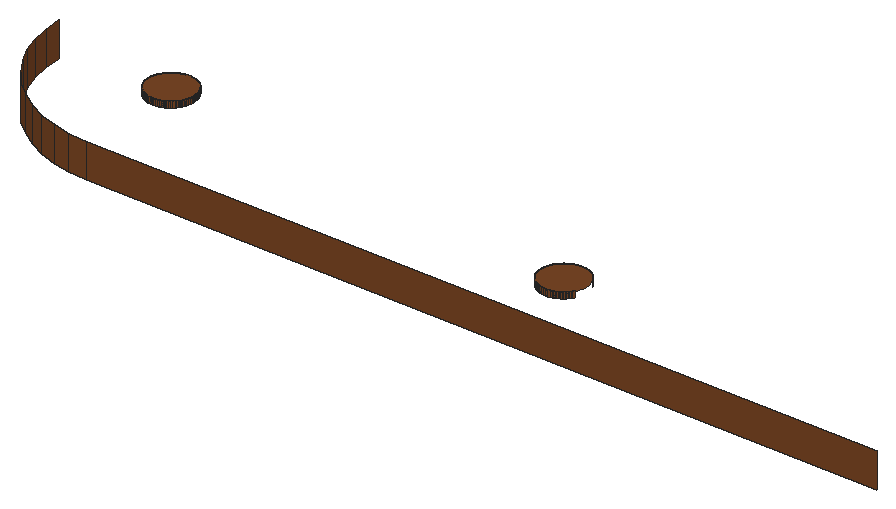
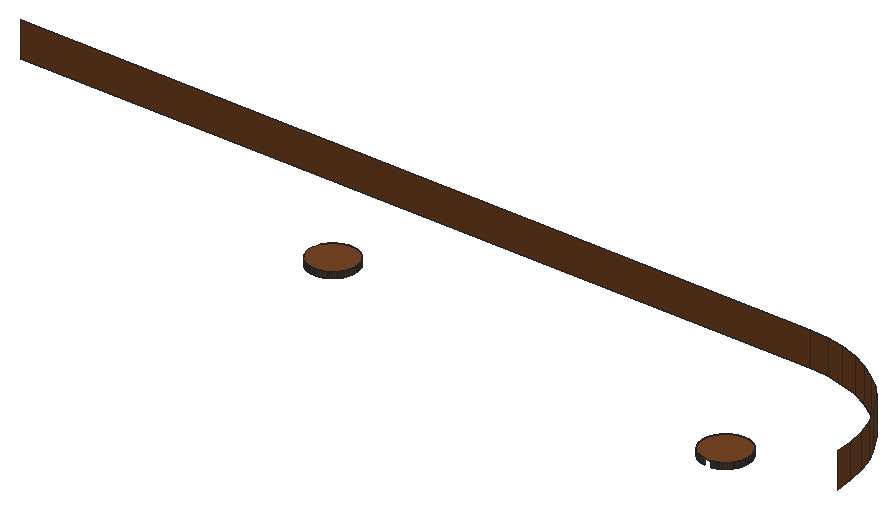
# SketchUp Ruby script. Lengths in inches.
U = 1.inch
M = Sketchup.active_model
def pt(a) = Geom::Point3d.new(a.map { |v| v * U })
def face(e, loops, mat)
  f = e.add_face(loops[0].map { |a| pt(a) })
  loops[1..].each { |l| e.add_face(l.map { |a| pt(a) }).erase! }
  f.material = f.back_material = mat if mat
  f
end
# faces: each face lists its corners as indices into pts; further lists are holes
def faces(e, pts, list, mat = nil) = list.each { |f| face(e, (f[0].is_a?(Array) ? f : [f]).map { |l| l.map { |i| pts[i] } }, mat) }
# xy, xz, yz: faces in a plane at the given z, y or x. An outline is a flat list of corners, or four numbers for a rectangle; further outlines are holes
def ring(l) = l.size == 4 ? [[l[0], l[1]], [l[2], l[1]], [l[2], l[3]], [l[0], l[3]]] : l.each_slice(2).to_a
def flat(e, list, mat, &to3) = list.each { |f| face(e, (f[0].is_a?(Array) ? f : [f]).map { |l| ring(l).map { |u, v| to3.(u, v) } }, mat) }
def xy(e, z, list, mat = nil) = flat(e, list, mat) { |x, y| [x, y, z] }
def xz(e, y, list, mat = nil) = flat(e, list, mat) { |x, z| [x, y, z] }
def yz(e, x, list, mat = nil) = flat(e, list, mat) { |y, z| [x, y, z] }
def lines(e, pts, list) = list.each { |a, b| e.add_line(pt(pts[a]), pt(pts[b])) }
# prism: a flat outline (further loops are holes) pulled along v
def prism(e, loops, v, mat = nil)
  f = face(e, loops, mat); d = Geom::Vector3d.new(v.map { |x| x * U })
  f.pushpull(f.normal.samedirection?(d) ? d.length : -d.length)
end
def box(e, o, s, mat = nil) = prism(e, [[o, [o[0] + s[0], o[1], o[2]], [o[0] + s[0], o[1] + s[1], o[2]], [o[0], o[1] + s[1], o[2]]]], [0, 0, s[2]], mat)
def at(x, y, z, deg = 0) = Geom::Transformation.translation(pt([x, y, z])) * Geom::Transformation.rotation(ORIGIN, Z_AXIS, deg.degrees)
def axes(o, x, y, z) = Geom::Transformation.new([*x, 0, *y, 0, *z, 0, *pt(o).to_a, 1])
def part(name) = M.definitions.add(name)
# library, detail: a bought-in or finely detailed component or shape, given as its bounding box
def library(name, o, s) = part(name).tap { |d| box(d.entities, o, s) }
def detail(e, o, s) = box(e.add_group.entities, o, s)
def put(e, d, t, mat = nil) = e.add_instance(d, t).tap { |i| i.material = mat if mat }
def group(e, t, mat = nil) = e.add_group.tap { |g| g.transformation = t; g.material = mat if mat }.entities
root = M.entities
M.materials.add("[Wood Veneer 01]3").color = [120, 70, 37]
xy(root,118.5,[[109.4,34,109.24,34.02,109.15,34.03,108.91,34.09,108.67,34.18,108.6,34.21,108.52,34.25,108.45,34.3,108.38,34.34,108.3125,34.39,108.25,34.44,108.18,34.5,108.12,34.55,108.0625,34.61,108,34.67,107.95,34.74,107.9,34.8,107.8,34.94,107.76,35.01,107.72,35.09,107.68,35.16,107.59,35.4,107.53,35.64,107.51,35.8,107.5,35.89,107.5,36.14,107.51,36.22,107.52,36.31,107.6,36.63,107.66,36.79,107.7,36.86,107.73,36.9375,107.77,37.01,107.97,37.29,108.02,37.35,108.14,37.47,108.2,37.52,108.27,37.58,108.34,37.625,108.4,37.67,108.48,37.72,108.55,37.76,108.625,37.8,108.7,37.83,108.94,37.92,109.1,37.96,109.18,37.97,109.26,37.99,109.35,37.99,109.43,38,109.6,38,109.76,37.98,109.85,37.97,110.09,37.91,110.33,37.82,110.4,37.79,110.48,37.75,110.55,37.7,110.62,37.66,110.6875,37.61,110.75,37.56,110.82,37.5,110.88,37.45,110.9375,37.39,111,37.33,111.05,37.26,111.1,37.2,111.2,37.06,111.24,36.99,111.28,36.91,111.32,36.84,111.41,36.6,111.47,36.36,111.49,36.2,111.5,36.11,111.5,35.86,111.49,35.78,111.48,35.69,111.4,35.37,111.34,35.21,111.3,35.14,111.27,35.0625,111.23,34.99,111.03,34.71,110.98,34.65,110.86,34.53,110.8,34.48,110.73,34.42,110.66,34.375,110.6,34.33,110.52,34.28,110.45,34.24,110.375,34.2,110.3,34.17,110.06,34.08,109.9,34.04,109.82,34.03,109.74,34.01,109.65,34.01,109.57,34],[71.9,38,71.74,38.02,71.65,38.03,71.41,38.09,71.17,38.18,71.1,38.21,71.02,38.25,70.95,38.3,70.88,38.34,70.8125,38.39,70.75,38.44,70.68,38.5,70.62,38.55,70.5625,38.61,70.5,38.67,70.45,38.74,70.4,38.8,70.3,38.94,70.26,39.01,70.22,39.09,70.18,39.16,70.09,39.4,70.03,39.64,70.01,39.8,70,39.89,70,40.14,70.01,40.22,70.02,40.31,70.1,40.63,70.16,40.79,70.2,40.86,70.23,40.9375,70.27,41.01,70.47,41.29,70.52,41.35,70.64,41.47,70.7,41.52,70.77,41.58,70.84,41.625,70.9,41.67,70.98,41.72,71.05,41.76,71.125,41.8,71.2,41.83,71.44,41.92,71.6,41.96,71.68,41.97,71.76,41.99,71.85,41.99,71.93,42,72.1,42,72.26,41.98,72.35,41.97,72.59,41.91,72.83,41.82,72.9,41.79,72.98,41.75,73.05,41.7,73.12,41.66,73.1875,41.61,73.25,41.56,73.32,41.5,73.38,41.45,73.4375,41.39,73.5,41.33,73.55,41.26,73.6,41.2,73.7,41.06,73.74,40.99,73.78,40.91,73.82,40.84,73.91,40.6,73.97,40.36,73.99,40.2,74,40.11,74,39.86,73.99,39.78,73.98,39.69,73.9,39.37,73.84,39.21,73.8,39.14,73.77,39.0625,73.73,38.99,73.53,38.71,73.48,38.65,73.36,38.53,73.3,38.48,73.23,38.42,73.16,38.375,73.1,38.33,73.02,38.28,72.95,38.24,72.875,38.2,72.8,38.17,72.56,38.08,72.4,38.04,72.32,38.03,72.24,38.01,72.15,38.01,72.07,38]],"[Wood Veneer 01]3")
xz(root,27,[[75,118,144,121]],"[Wood Veneer 01]3")
xz(root,34,[[109.4,118,109.49,118.5],[109.49,118,109.57,118.5]],"[Wood Veneer 01]3")
xz(root,34.01,[[109.65,118,109.74,118.5]],"[Wood Veneer 01]3")
xz(root,37.99,[[109.26,118,109.35,118.5]],"[Wood Veneer 01]3")
xz(root,38,[[71.9,118,71.99,118.5],[71.99,118,72.07,118.5],[109.43,118,109.51,118.5],[109.51,118,109.6,118.5]],"[Wood Veneer 01]3")
xz(root,38.01,[[72.15,118,72.24,118.5]],"[Wood Veneer 01]3")
yz(root,70,[[39.89,118,39.97,118.5],[39.97,118,40.06,118.5],[40.06,118,40.14,118.5]],"[Wood Veneer 01]3")
yz(root,74,[[39.86,118,39.94,118.5],[39.94,118,40.03,118.5],[40.03,118,40.11,118.5]],"[Wood Veneer 01]3")
yz(root,107.5,[[35.89,118,35.97,118.5],[35.97,118,36.06,118.5],[36.06,118,36.14,118.5]],"[Wood Veneer 01]3")
p = [[75,27,121],[73.43,27.1,121],[73.43,27.1,118],[75,27,118],[71.89,27.41,121],[71.89,27.41,118],
  [70.41,27.91,121],[70.41,27.91,118],[69,28.61,121],[69,28.61,118],[67.69,29.48,121],[67.69,29.48,118],
  [66.51,30.51,121],[66.51,30.51,118],[65.48,31.69,121],[65.48,31.69,118],[64.61,33,121],[64.61,33,118],
  [63.91,34.41,121],[63.91,34.41,118],[109.07,34.05,118],[108.99,34.07,118],[108.99,34.07,118.5],[109.07,34.05,118.5],
  [109.15,34.03,118],[109.15,34.03,118.5],[109.32,34.01,118],[109.24,34.02,118],[109.24,34.02,118.5],[109.32,34.01,118.5],
  [109.4,34,118],[109.4,34,118.5],[109.65,34.01,118],[109.57,34,118],[109.57,34,118.5],[109.65,34.01,118.5],
  [109.82,34.03,118],[109.74,34.01,118],[109.74,34.01,118.5],[109.82,34.03,118.5],[109.9,34.04,118],[109.9,34.04,118.5],
  [109.98,34.06,118],[109.98,34.06,118.5],[108.75,34.15,118],[108.67,34.18,118],[108.67,34.18,118.5],[108.75,34.15,118.5],
  [108.91,34.09,118],[108.83,34.12,118],[108.83,34.12,118.5],[108.91,34.09,118.5],[110.06,34.08,118],[110.06,34.08,118.5],
  [110.14,34.11,118],[110.14,34.11,118.5],[110.22,34.14,118],[110.22,34.14,118.5],[110.3,34.17,118],[110.3,34.17,118.5],
  [108.6,34.21,118],[108.52,34.25,118],[108.52,34.25,118.5],[108.6,34.21,118.5],[110.375,34.2,118],[110.375,34.2,118.5],
  [110.45,34.24,118],[110.45,34.24,118.5],[110.52,34.28,118],[110.52,34.28,118.5],[108.38,34.34,118],[108.3125,34.39,118],
  [108.3125,34.39,118.5],[108.38,34.34,118.5],[108.45,34.3,118],[108.45,34.3,118.5],[110.6,34.33,118],[110.6,34.33,118.5],
  [110.66,34.375,118],[110.66,34.375,118.5],[63.41,35.89,121],[63.41,35.89,118],[108.25,34.44,118],[108.25,34.44,118.5],
  [108.18,34.5,118],[108.18,34.5,118.5],[110.73,34.42,118],[110.73,34.42,118.5],[110.8,34.48,118],[110.8,34.48,118.5],
  [108.12,34.55,118],[108.12,34.55,118.5],[110.86,34.53,118],[110.86,34.53,118.5],[110.92,34.59,118],[110.92,34.59,118.5],
  [108.0625,34.61,118],[108,34.67,118],[108,34.67,118.5],[108.0625,34.61,118.5],[110.98,34.65,118],[110.98,34.65,118.5],
  [107.95,34.74,118],[107.9,34.8,118],[107.9,34.8,118.5],[107.95,34.74,118.5],[111.03,34.71,118],[111.03,34.71,118.5],
  [111.08,34.78,118],[111.08,34.78,118.5],[107.85,34.87,118],[107.85,34.87,118.5],[111.13,34.85,118],[111.13,34.85,118.5],
  [111.18,34.92,118],[111.18,34.92,118.5],[107.8,34.94,118],[107.8,34.94,118.5],[107.76,35.01,118],[107.76,35.01,118.5],
  [111.23,34.99,118],[111.23,34.99,118.5],[107.72,35.09,118],[107.72,35.09,118.5],[107.68,35.16,118],[107.68,35.16,118.5],
  [107.65,35.24,118],[107.62,35.32,118],[107.62,35.32,118.5],[107.65,35.24,118.5],[107.59,35.4,118],[107.59,35.4,118.5],
  [107.57,35.48,118],[107.57,35.48,118.5],[107.55,35.56,118],[107.55,35.56,118.5],[107.53,35.64,118],[107.53,35.64,118.5],
  [107.52,35.72,118],[107.52,35.72,118.5],[107.51,35.8,118],[107.51,35.8,118.5],[107.5,35.89,118],[107.5,35.89,118.5],
  [63.1,37.43,121],[63.1,37.43,118],[107.5,36.14,118],[107.51,36.22,118],[107.51,36.22,118.5],[107.5,36.14,118.5],
  [107.52,36.31,118],[107.52,36.31,118.5],[107.54,36.39,118],[107.54,36.39,118.5],[107.56,36.47,118],[107.56,36.47,118.5],
  [107.58,36.55,118],[107.58,36.55,118.5],[107.6,36.63,118],[107.6,36.63,118.5],[107.63,36.71,118],[107.63,36.71,118.5],
  [107.66,36.79,118],[107.66,36.79,118.5],[107.7,36.86,118],[107.7,36.86,118.5],[107.73,36.9375,118],[107.73,36.9375,118.5],
  [107.77,37.01,118],[107.77,37.01,118.5],[107.82,37.08,118],[107.82,37.08,118.5],[111.2,37.06,118],[111.24,36.99,118],
  [111.24,36.99,118.5],[111.2,37.06,118.5],[107.87,37.15,118],[107.87,37.15,118.5],[111.1,37.2,118],[111.15,37.13,118],
  [111.15,37.13,118.5],[111.1,37.2,118.5],[107.92,37.22,118],[107.92,37.22,118.5],[107.97,37.29,118],[107.97,37.29,118.5],
  [111.05,37.26,118],[111.05,37.26,118.5],[108.02,37.35,118],[108.02,37.35,118.5],[108.08,37.41,118],[108.08,37.41,118.5],
  [110.9375,37.39,118],[111,37.33,118],[111,37.33,118.5],[110.9375,37.39,118.5],[63,39,121],[63,39,118],
  [108.14,37.47,118],[108.14,37.47,118.5],[110.82,37.5,118],[110.88,37.45,118],[110.88,37.45,118.5],[110.82,37.5,118.5],
  [108.2,37.52,118],[108.2,37.52,118.5],[108.27,37.58,118],[108.27,37.58,118.5],[110.75,37.56,118],[110.75,37.56,118.5],
  [108.34,37.625,118],[108.34,37.625,118.5],[108.4,37.67,118],[108.4,37.67,118.5],[110.62,37.66,118],[110.6875,37.61,118],
  [110.6875,37.61,118.5],[110.62,37.66,118.5],[108.48,37.72,118],[108.48,37.72,118.5],[108.55,37.76,118],[108.55,37.76,118.5],
  [110.4,37.79,118],[110.48,37.75,118],[110.48,37.75,118.5],[110.4,37.79,118.5],[110.55,37.7,118],[110.55,37.7,118.5],
  [108.625,37.8,118],[108.625,37.8,118.5],[108.7,37.83,118],[108.7,37.83,118.5],[108.78,37.86,118],[108.78,37.86,118.5],
  [110.25,37.85,118],[110.33,37.82,118],[110.33,37.82,118.5],[110.25,37.85,118.5],[108.86,37.89,118],[108.86,37.89,118.5],
  [108.94,37.92,118],[108.94,37.92,118.5],[109.02,37.94,118],[109.02,37.94,118.5],[109.1,37.96,118],[109.1,37.96,118.5],
  [109.93,37.95,118],[110.01,37.93,118],[110.01,37.93,118.5],[109.93,37.95,118.5],[110.09,37.91,118],[110.09,37.91,118.5],
  [110.17,37.88,118],[110.17,37.88,118.5],[71.57,38.05,118],[71.49,38.07,118],[71.49,38.07,118.5],[71.57,38.05,118.5],
  [71.65,38.03,118],[71.65,38.03,118.5],[71.82,38.01,118],[71.74,38.02,118],[71.74,38.02,118.5],[71.82,38.01,118.5],
  [71.9,38,118],[71.9,38,118.5],[72.15,38.01,118],[72.07,38,118],[72.07,38,118.5],[72.15,38.01,118.5],
  [72.32,38.03,118],[72.24,38.01,118],[72.24,38.01,118.5],[72.32,38.03,118.5],[72.4,38.04,118],[72.4,38.04,118.5],
  [72.48,38.06,118],[72.48,38.06,118.5],[109.18,37.97,118],[109.18,37.97,118.5],[109.26,37.99,118],[109.26,37.99,118.5],
  [109.35,37.99,118],[109.43,38,118],[109.43,38,118.5],[109.35,37.99,118.5],[109.6,38,118],[109.68,37.99,118],
  [109.68,37.99,118.5],[109.6,38,118.5],[109.76,37.98,118],[109.76,37.98,118.5],[109.85,37.97,118],[109.85,37.97,118.5],
  [71.25,38.15,118],[71.17,38.18,118],[71.17,38.18,118.5],[71.25,38.15,118.5],[71.41,38.09,118],[71.33,38.12,118],
  [71.33,38.12,118.5],[71.41,38.09,118.5],[72.56,38.08,118],[72.56,38.08,118.5],[72.64,38.11,118],[72.64,38.11,118.5],
  [72.72,38.14,118],[72.72,38.14,118.5],[72.8,38.17,118],[72.8,38.17,118.5],[71.1,38.21,118],[71.02,38.25,118],
  [71.02,38.25,118.5],[71.1,38.21,118.5],[72.875,38.2,118],[72.875,38.2,118.5],[72.95,38.24,118],[72.95,38.24,118.5],
  [73.02,38.28,118],[73.02,38.28,118.5],[70.88,38.34,118],[70.8125,38.39,118],[70.8125,38.39,118.5],[70.88,38.34,118.5],
  [70.95,38.3,118],[70.95,38.3,118.5],[73.1,38.33,118],[73.1,38.33,118.5],[73.16,38.375,118],[73.16,38.375,118.5],
  [70.75,38.44,118],[70.75,38.44,118.5],[70.68,38.5,118],[70.68,38.5,118.5],[73.23,38.42,118],[73.23,38.42,118.5],
  [73.3,38.48,118],[73.3,38.48,118.5],[70.62,38.55,118],[70.62,38.55,118.5],[73.36,38.53,118],[73.36,38.53,118.5],
  [73.42,38.59,118],[73.42,38.59,118.5],[70.5625,38.61,118],[70.5,38.67,118],[70.5,38.67,118.5],[70.5625,38.61,118.5],
  [73.48,38.65,118],[73.48,38.65,118.5],[70.45,38.74,118],[70.4,38.8,118],[70.4,38.8,118.5],[70.45,38.74,118.5],
  [73.53,38.71,118],[73.53,38.71,118.5],[73.58,38.78,118],[73.58,38.78,118.5],[70.35,38.87,118],[70.35,38.87,118.5],
  [73.63,38.85,118],[73.63,38.85,118.5],[73.68,38.92,118],[73.68,38.92,118.5],[70.3,38.94,118],[70.3,38.94,118.5],
  [70.26,39.01,118],[70.26,39.01,118.5],[73.73,38.99,118],[73.73,38.99,118.5],[70.22,39.09,118],[70.22,39.09,118.5],
  [73.77,39.0625,118],[73.77,39.0625,118.5],[70.18,39.16,118],[70.18,39.16,118.5],[73.8,39.14,118],[73.8,39.14,118.5],
  [73.84,39.21,118],[73.84,39.21,118.5],[70.15,39.24,118],[70.12,39.32,118],[70.12,39.32,118.5],[70.15,39.24,118.5],
  [73.87,39.29,118],[73.87,39.29,118.5],[70.09,39.4,118],[70.09,39.4,118.5],[73.9,39.37,118],[73.9,39.37,118.5],
  [70.07,39.48,118],[70.07,39.48,118.5],[73.92,39.45,118],[73.92,39.45,118.5],[73.94,39.53,118],[73.94,39.53,118.5],
  [70.05,39.56,118],[70.05,39.56,118.5],[73.96,39.61,118],[73.96,39.61,118.5],[70.03,39.64,118],[70.03,39.64,118.5],
  [70.02,39.72,118],[70.02,39.72,118.5],[73.98,39.69,118],[73.98,39.69,118.5],[70.01,39.8,118],[70.01,39.8,118.5],
  [73.99,39.78,118],[73.99,39.78,118.5],[70,39.89,118],[70,39.89,118.5],[74,39.86,118],[74,39.86,118.5],
  [70,40.14,118],[70.01,40.22,118],[70.01,40.22,118.5],[70,40.14,118.5],[73.99,40.2,118],[74,40.11,118],
  [74,40.11,118.5],[73.99,40.2,118.5],[70.02,40.31,118],[70.02,40.31,118.5],[73.98,40.28,118],[73.98,40.28,118.5],
  [70.04,40.39,118],[70.04,40.39,118.5],[73.97,40.36,118],[73.97,40.36,118.5],[70.06,40.47,118],[70.06,40.47,118.5],
  [73.93,40.52,118],[73.95,40.44,118],[73.95,40.44,118.5],[73.93,40.52,118.5],[70.08,40.55,118],[70.08,40.55,118.5],
  [73.91,40.6,118],[73.91,40.6,118.5],[70.1,40.63,118],[70.1,40.63,118.5],[70.13,40.71,118],[70.13,40.71,118.5],
  [73.88,40.68,118],[73.88,40.68,118.5],[70.16,40.79,118],[70.16,40.79,118.5],[73.85,40.76,118],[73.85,40.76,118.5],
  [70.2,40.86,118],[70.2,40.86,118.5],[73.82,40.84,118],[73.82,40.84,118.5],[73.78,40.91,118],[73.78,40.91,118.5],
  [70.23,40.9375,118],[70.23,40.9375,118.5],[70.27,41.01,118],[70.27,41.01,118.5],[73.74,40.99,118],[73.74,40.99,118.5],
  [70.32,41.08,118],[70.32,41.08,118.5],[73.7,41.06,118],[73.7,41.06,118.5],[70.37,41.15,118],[70.37,41.15,118.5],
  [73.6,41.2,118],[73.65,41.13,118],[73.65,41.13,118.5],[73.6,41.2,118.5],[70.42,41.22,118],[70.42,41.22,118.5],
  [70.47,41.29,118],[70.47,41.29,118.5],[73.55,41.26,118],[73.55,41.26,118.5],[70.52,41.35,118],[70.52,41.35,118.5],
  [70.58,41.41,118],[70.58,41.41,118.5],[73.4375,41.39,118],[73.5,41.33,118],[73.5,41.33,118.5],[73.4375,41.39,118.5],
  [70.64,41.47,118],[70.64,41.47,118.5],[73.32,41.5,118],[73.38,41.45,118],[73.38,41.45,118.5],[73.32,41.5,118.5],
  [70.7,41.52,118],[70.7,41.52,118.5],[70.77,41.58,118],[70.77,41.58,118.5],[73.25,41.56,118],[73.25,41.56,118.5],
  [70.84,41.625,118],[70.84,41.625,118.5],[70.9,41.67,118],[70.9,41.67,118.5],[73.12,41.66,118],[73.1875,41.61,118],
  [73.1875,41.61,118.5],[73.12,41.66,118.5],[70.98,41.72,118],[70.98,41.72,118.5],[71.05,41.76,118],[71.05,41.76,118.5],
  [72.9,41.79,118],[72.98,41.75,118],[72.98,41.75,118.5],[72.9,41.79,118.5],[73.05,41.7,118],[73.05,41.7,118.5],
  [71.125,41.8,118],[71.125,41.8,118.5],[71.2,41.83,118],[71.2,41.83,118.5],[71.28,41.86,118],[71.28,41.86,118.5],
  [72.75,41.85,118],[72.83,41.82,118],[72.83,41.82,118.5],[72.75,41.85,118.5],[71.36,41.89,118],[71.36,41.89,118.5],
  [71.44,41.92,118],[71.44,41.92,118.5],[71.52,41.94,118],[71.52,41.94,118.5],[71.6,41.96,118],[71.6,41.96,118.5],
  [72.43,41.95,118],[72.51,41.93,118],[72.51,41.93,118.5],[72.43,41.95,118.5],[72.59,41.91,118],[72.59,41.91,118.5],
  [72.67,41.88,118],[72.67,41.88,118.5],[71.68,41.97,118],[71.68,41.97,118.5],[72.35,41.97,118],[72.35,41.97,118.5],
  [72.26,41.98,118],[72.26,41.98,118.5]]
faces(root,p,[[0,1,2,3],[1,4,5,2],[4,6,7,5],[6,8,9,7],[8,10,11,9],[10,12,13,11],[12,14,15,13],[14,16,17,15],
  [16,18,19,17],[20,21,22,23],[24,20,23,25],[26,27,28,29],[27,24,25,28],[30,26,29,31],[32,33,34,35],[36,37,38,39],
  [40,36,39,41],[42,40,41,43],[44,45,46,47],[48,49,50,51],[49,44,47,50],[21,48,51,22],[52,42,43,53],[54,52,53,55],
  [56,54,55,57],[58,56,57,59],[60,61,62,63],[45,60,63,46],[64,58,59,65],[66,64,65,67],[68,66,67,69],[70,71,72,73],
  [74,70,73,75],[61,74,75,62],[76,68,69,77],[78,76,77,79],[18,80,81,19],[71,82,83,72],[82,84,85,83],[86,78,79,87],
  [88,86,87,89],[84,90,91,85],[92,88,89,93],[94,92,93,95],[96,97,98,99],[90,96,99,91],[100,94,95,101],[102,103,104,105],
  [97,102,105,98],[106,100,101,107],[108,106,107,109],[103,110,111,104],[112,108,109,113],[114,112,113,115],[110,116,117,111],[116,118,119,117],
  [120,114,115,121],[118,122,123,119],[122,124,125,123],[126,127,128,129],[124,126,129,125],[127,130,131,128],[130,132,133,131],[132,134,135,133],
  [134,136,137,135],[136,138,139,137],[138,140,141,139],[140,142,143,141],[80,144,145,81],[146,147,148,149],[147,150,151,148],[150,152,153,151],
  [152,154,155,153],[154,156,157,155],[156,158,159,157],[158,160,161,159],[160,162,163,161],[162,164,165,163],[164,166,167,165],[166,168,169,167],
  [168,170,171,169],[172,173,174,175],[170,176,177,171],[178,179,180,181],[179,172,175,180],[176,182,183,177],[182,184,185,183],[186,178,181,187],
  [184,188,189,185],[188,190,191,189],[192,193,194,195],[193,186,187,194],[144,196,197,145],[190,198,199,191],[200,201,202,203],[201,192,195,202],
  [198,204,205,199],[204,206,207,205],[208,200,203,209],[206,210,211,207],[210,212,213,211],[214,215,216,217],[215,208,209,216],[212,218,219,213],
  [218,220,221,219],[222,223,224,225],[226,214,217,227],[223,226,227,224],[220,228,229,221],[228,230,231,229],[230,232,233,231],[234,235,236,237],
  [235,222,225,236],[232,238,239,233],[238,240,241,239],[240,242,243,241],[242,244,245,243],[246,247,248,249],[247,250,251,248],[250,252,253,251],
  [252,234,237,253],[254,255,256,257],[258,254,257,259],[260,261,262,263],[261,258,259,262],[264,260,263,265],[266,267,268,269],[270,271,272,273],
  [274,270,273,275],[276,274,275,277],[244,278,279,245],[278,280,281,279],[282,283,284,285],[286,287,288,289],[287,290,291,288],[292,246,249,293],
  [290,292,293,291],[294,295,296,297],[298,299,300,301],[299,294,297,300],[255,298,301,256],[302,276,277,303],[304,302,303,305],[306,304,305,307],
  [308,306,307,309],[310,311,312,313],[295,310,313,296],[314,308,309,315],[316,314,315,317],[318,316,317,319],[320,321,322,323],[324,320,323,325],
  [311,324,325,312],[326,318,319,327],[328,326,327,329],[321,330,331,322],[330,332,333,331],[334,328,329,335],[336,334,335,337],[332,338,339,333],
  [340,336,337,341],[342,340,341,343],[344,345,346,347],[338,344,347,339],[348,342,343,349],[350,351,352,353],[345,350,353,346],[354,348,349,355],
  [356,354,355,357],[351,358,359,352],[360,356,357,361],[362,360,361,363],[358,364,365,359],[364,366,367,365],[368,362,363,369],[366,370,371,367],
  [372,368,369,373],[370,374,375,371],[376,372,373,377],[378,376,377,379],[380,381,382,383],[374,380,383,375],[384,378,379,385],[381,386,387,382],
  [388,384,385,389],[386,390,391,387],[392,388,389,393],[394,392,393,395],[390,396,397,391],[398,394,395,399],[396,400,401,397],[400,402,403,401],
  [404,398,399,405],[402,406,407,403],[408,404,405,409],[406,410,411,407],[412,408,409,413],[414,415,416,417],[418,419,420,421],[415,422,423,416],
  [424,418,421,425],[422,426,427,423],[428,424,425,429],[426,430,431,427],[432,433,434,435],[433,428,429,434],[430,436,437,431],[438,432,435,439],
  [436,440,441,437],[440,442,443,441],[444,438,439,445],[442,446,447,443],[448,444,445,449],[446,450,451,447],[452,448,449,453],[454,452,453,455],
  [450,456,457,451],[456,458,459,457],[460,454,455,461],[458,462,463,459],[464,460,461,465],[462,466,467,463],[468,469,470,471],[469,464,465,470],
  [466,472,473,467],[472,474,475,473],[476,468,471,477],[474,478,479,475],[478,480,481,479],[482,483,484,485],[483,476,477,484],[480,486,487,481],
  [488,489,490,491],[489,482,485,490],[486,492,493,487],[492,494,495,493],[496,488,491,497],[494,498,499,495],[498,500,501,499],[502,503,504,505],
  [503,496,497,504],[500,506,507,501],[506,508,509,507],[510,511,512,513],[514,502,505,515],[511,514,515,512],[508,516,517,509],[516,518,519,517],
  [518,520,521,519],[522,523,524,525],[523,510,513,524],[520,526,527,521],[526,528,529,527],[528,530,531,529],[530,532,533,531],[534,535,536,537],
  [535,538,539,536],[538,540,541,539],[540,522,525,541],[532,542,543,533],[544,534,537,545],[546,544,545,547]],"[Wood Veneer 01]3")
